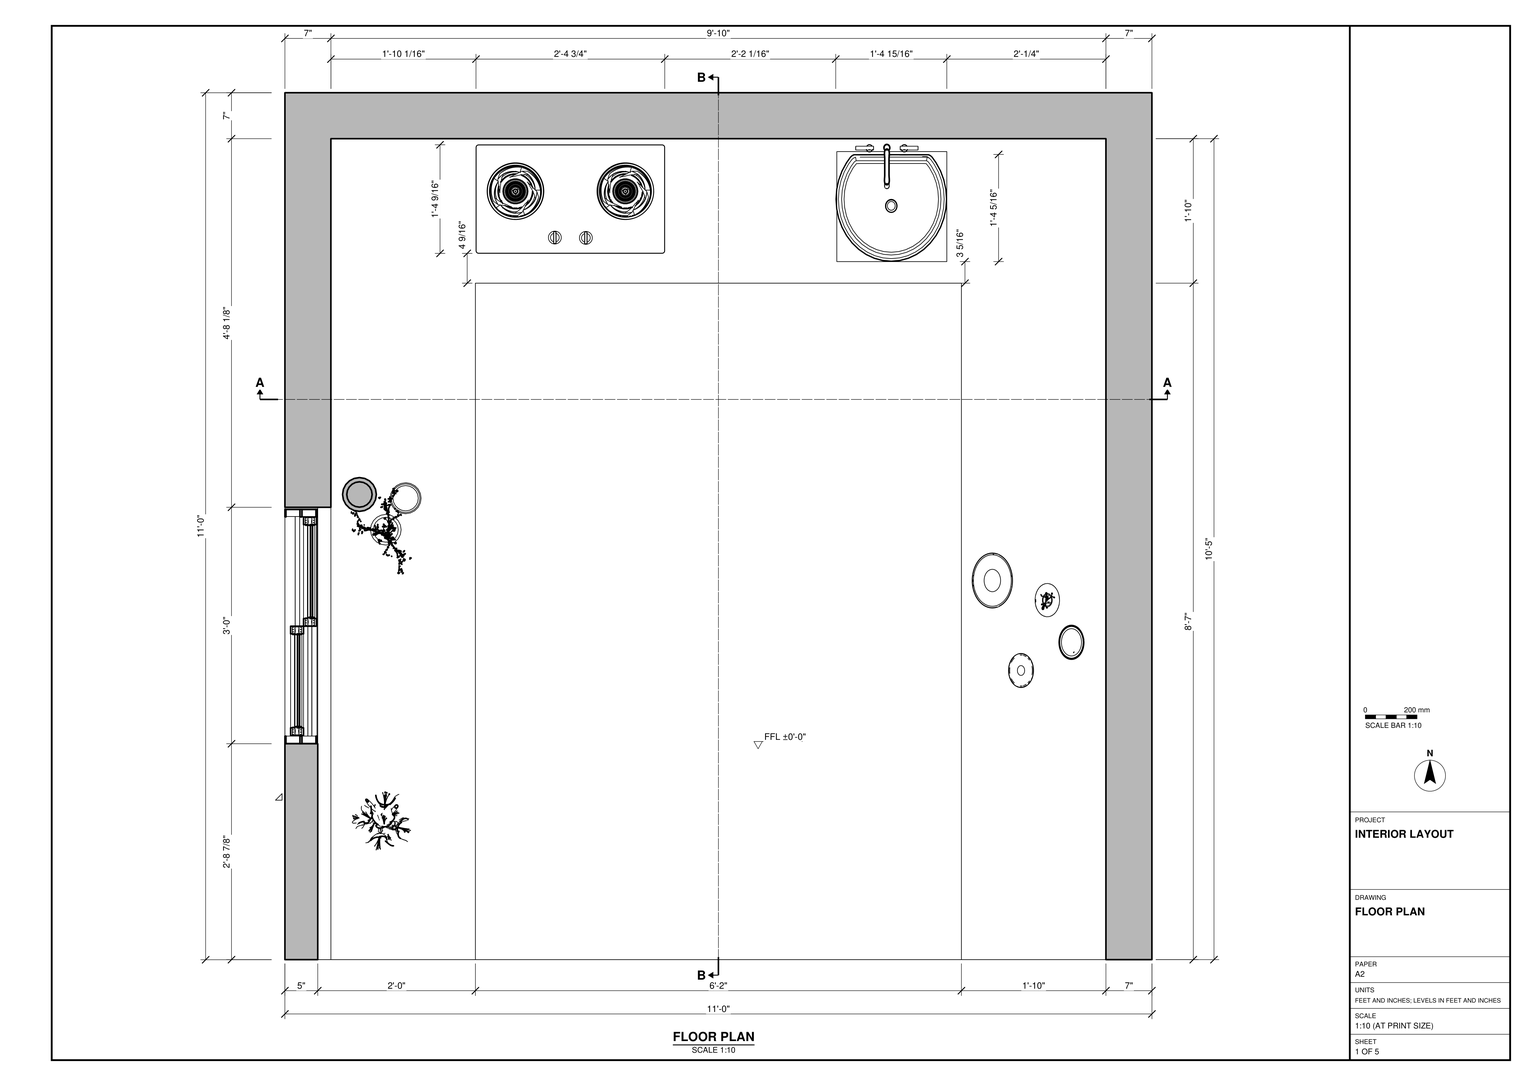
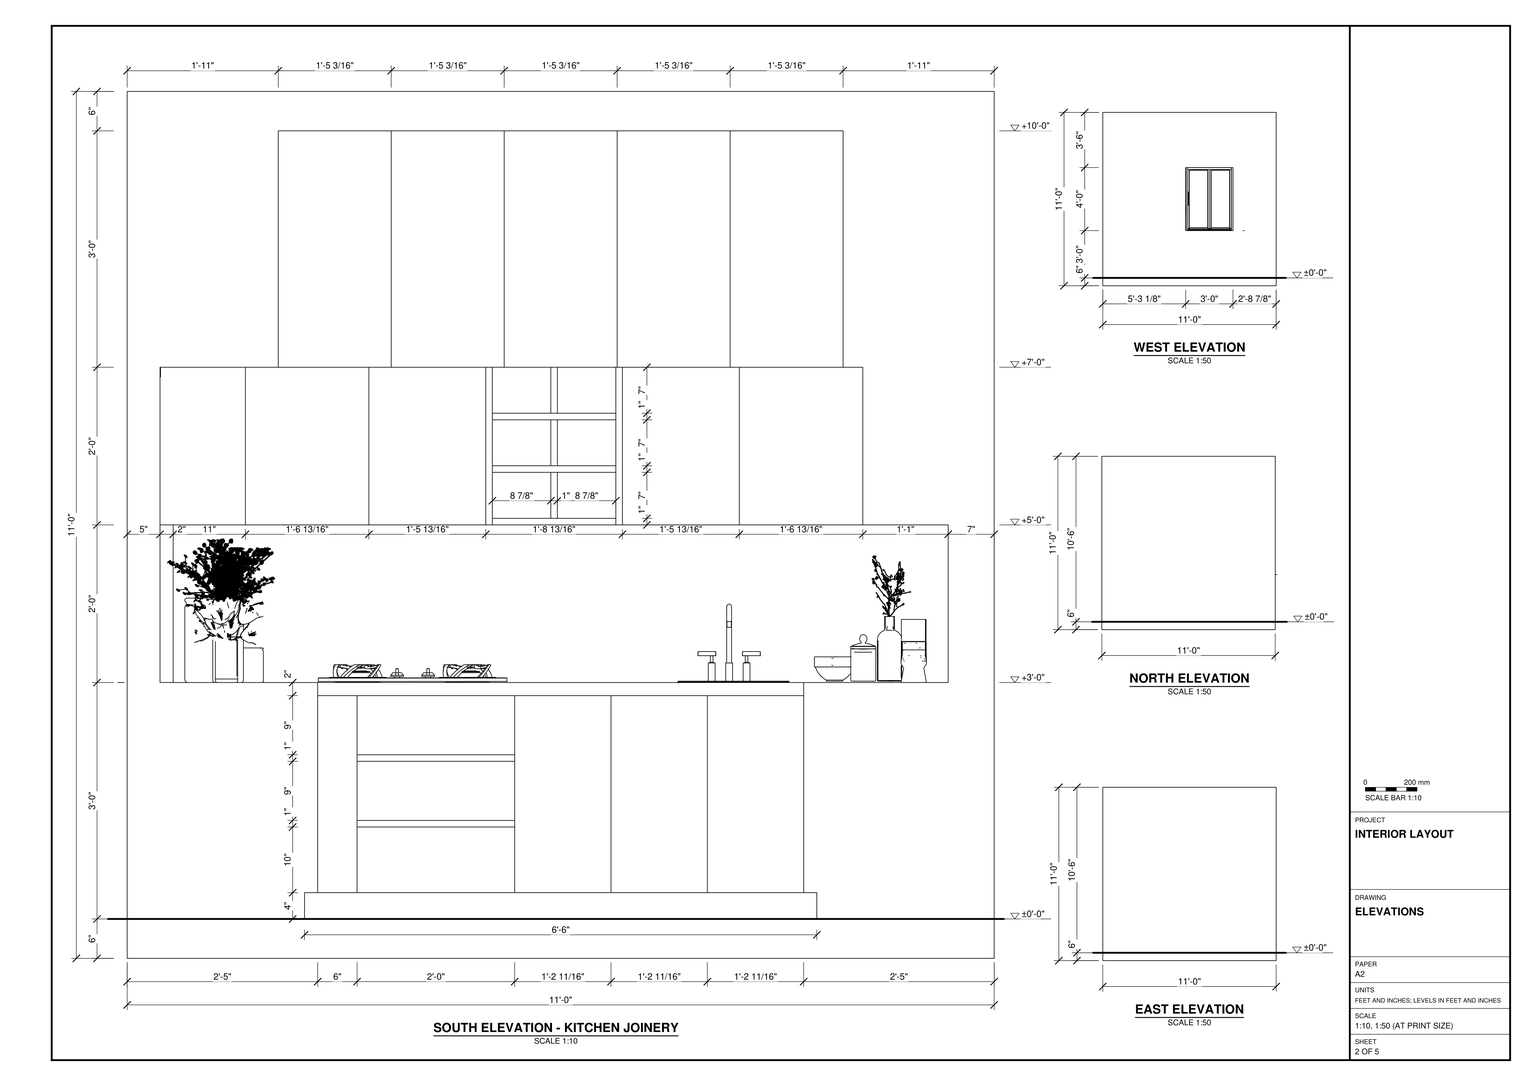
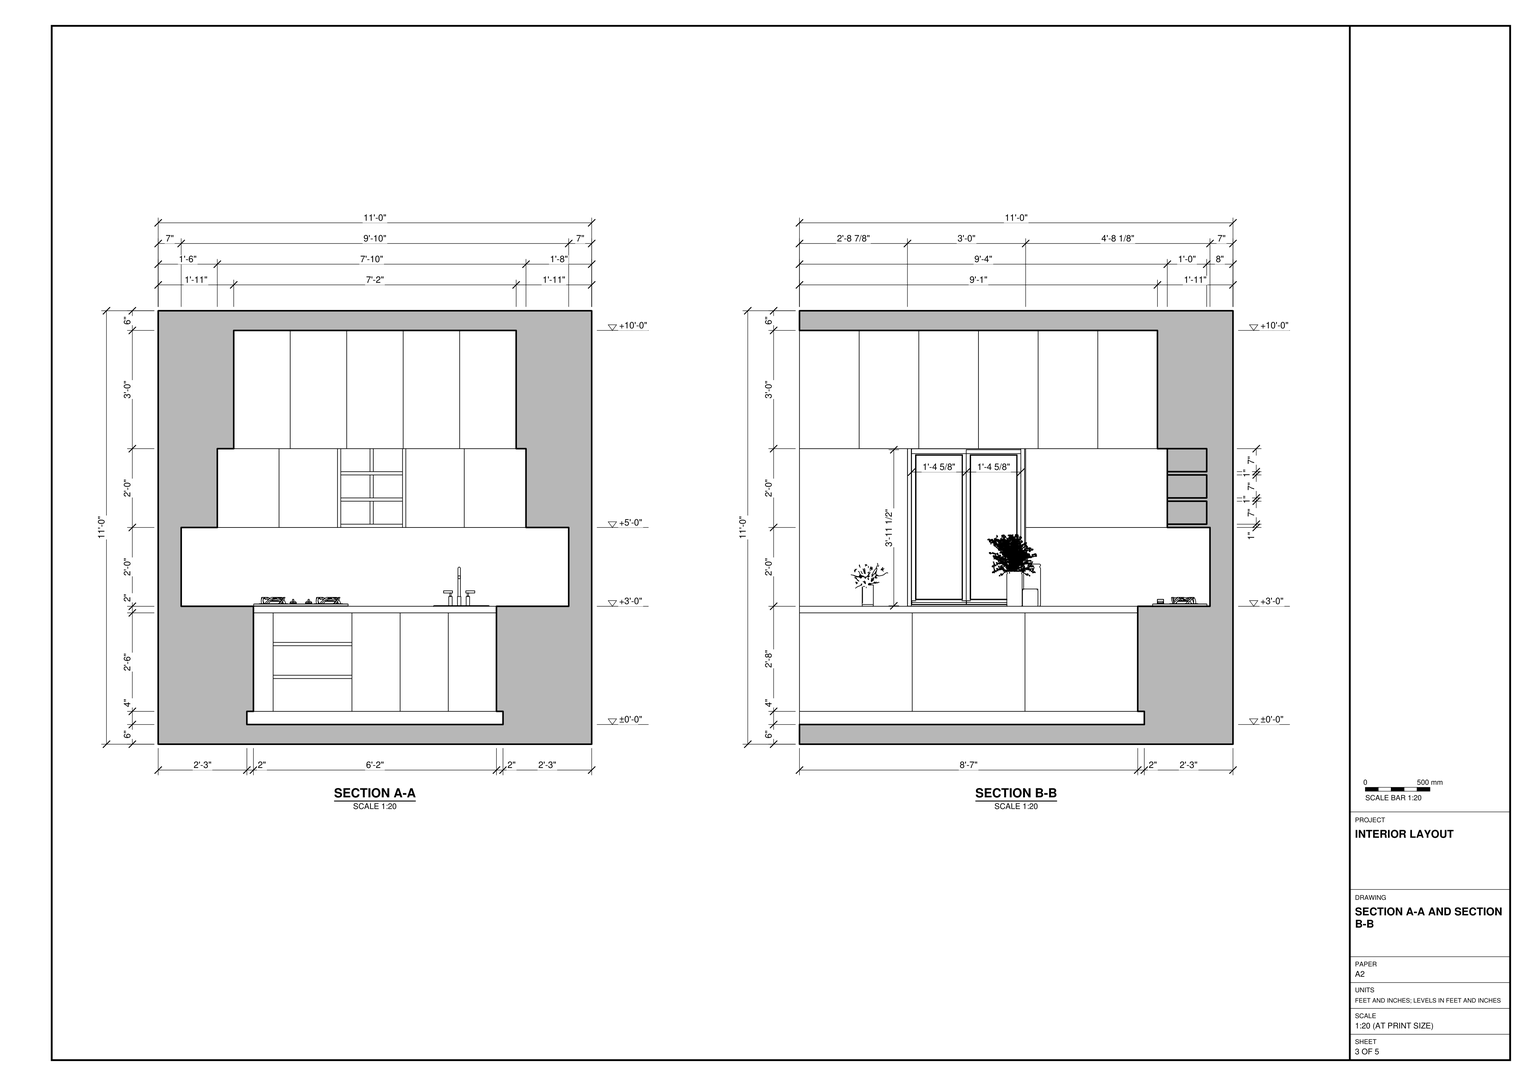
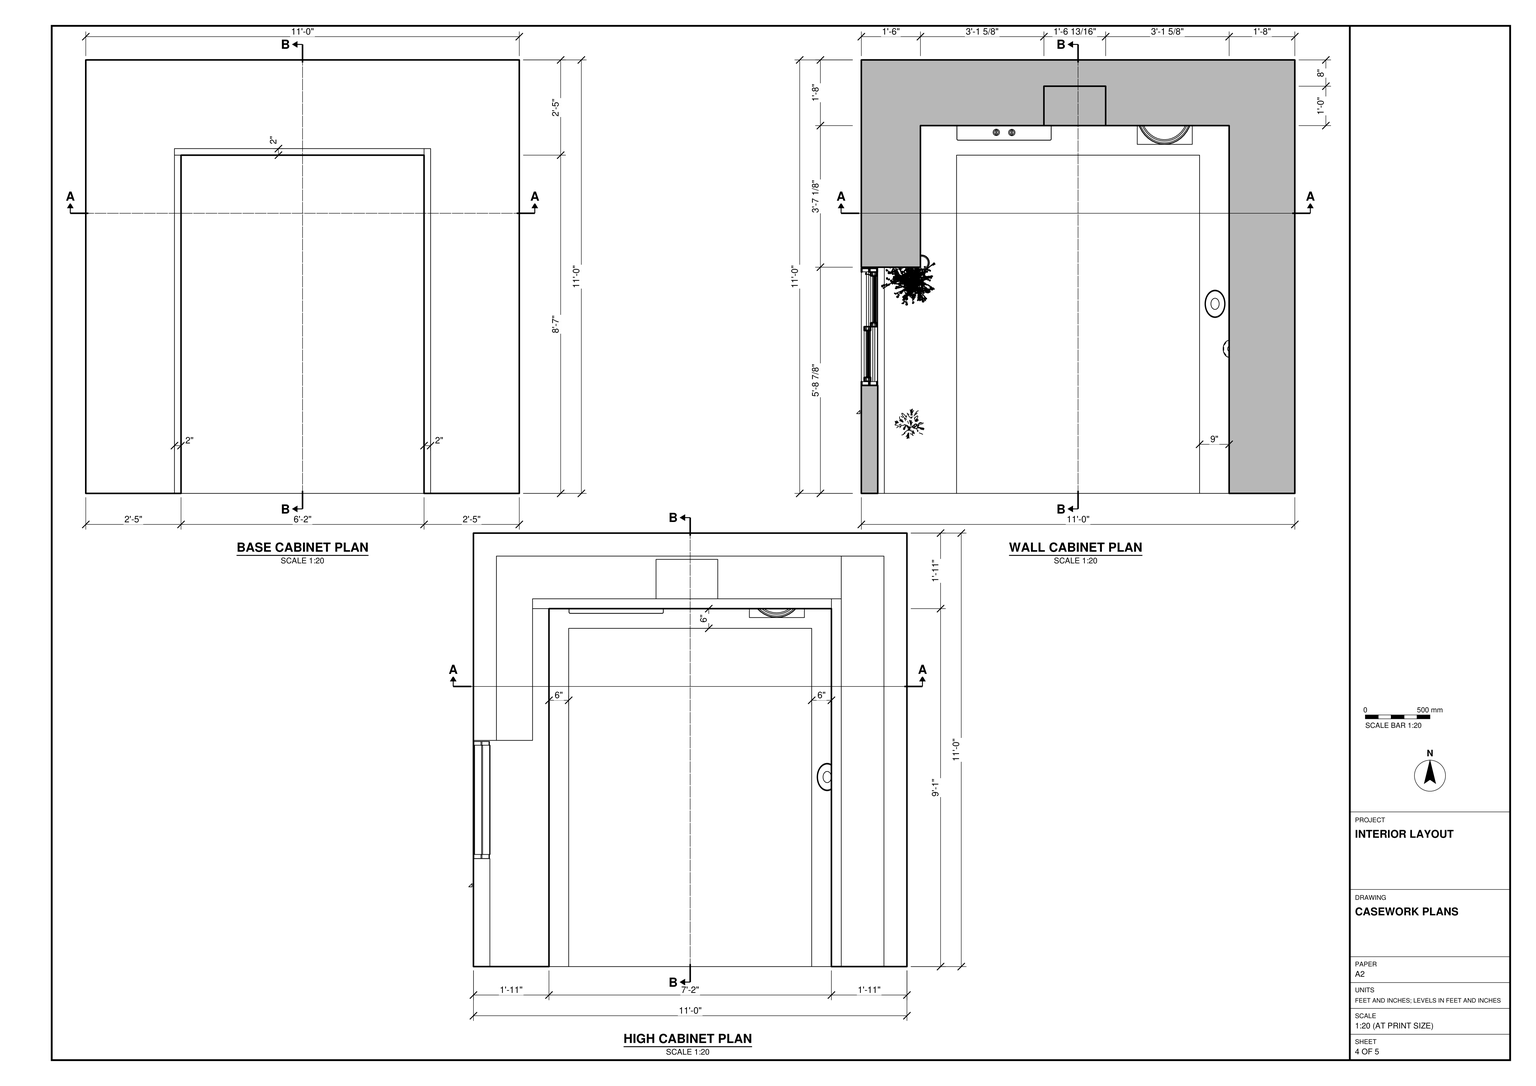
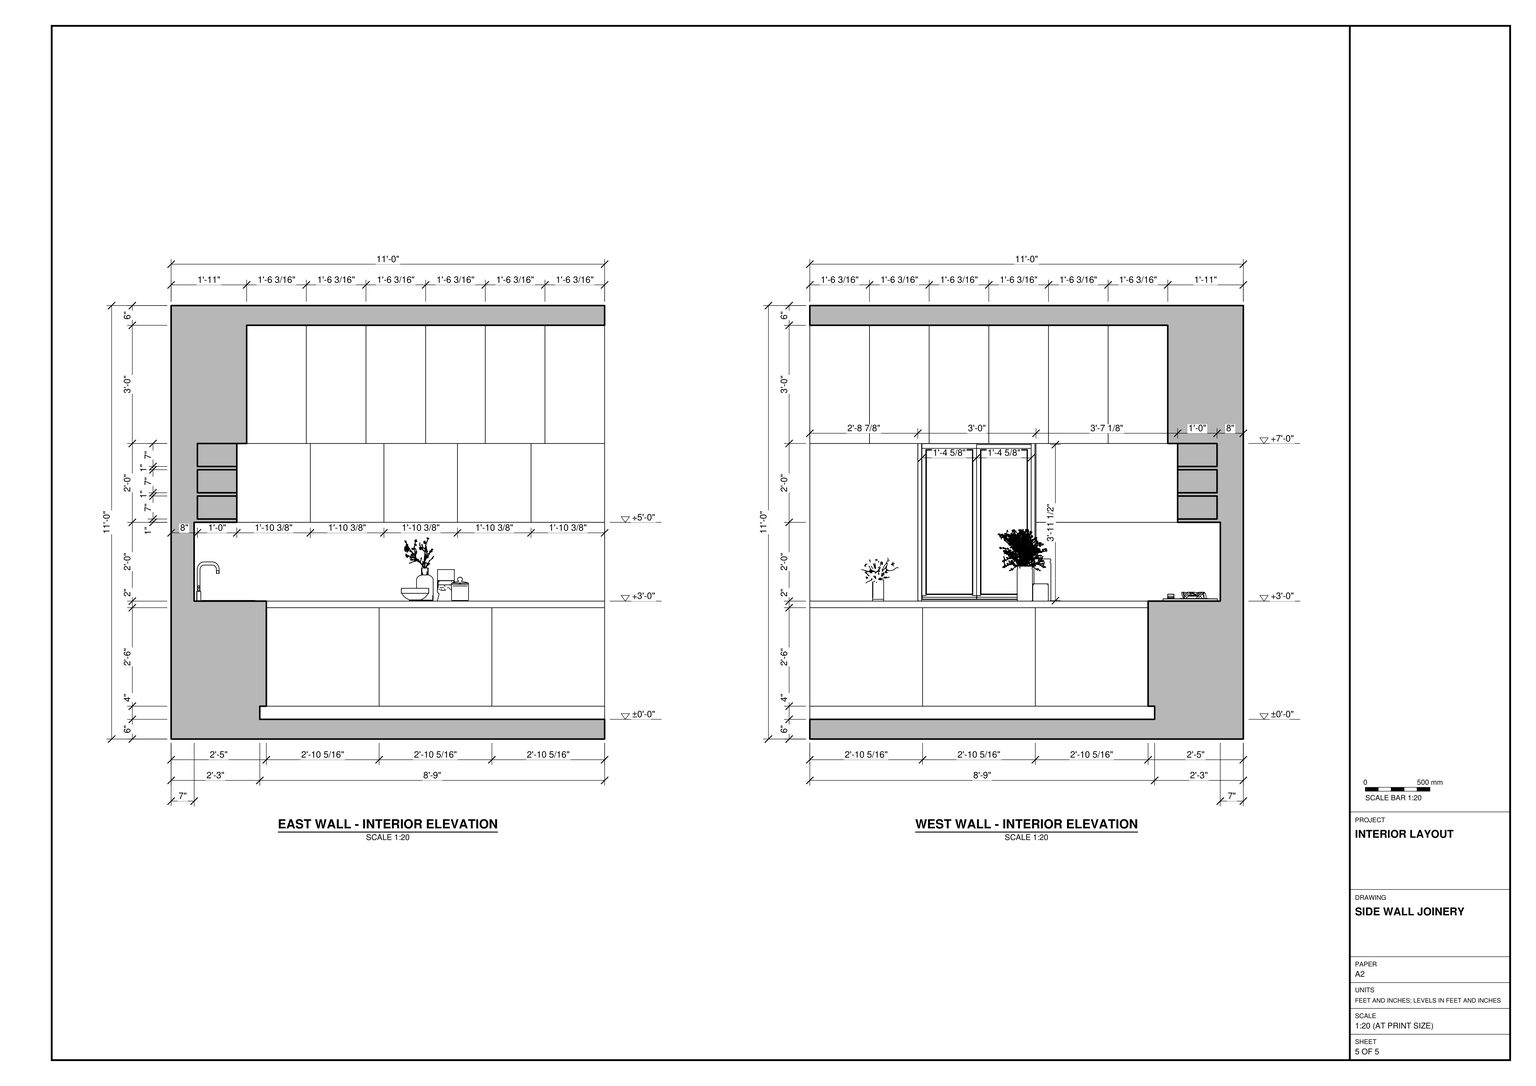
Build the kitchen interior in SketchUp using task_files/diagram_01.pdf. Work in feet and inches. The room is 11'-0" wide, 11'-0" deep and 11'-0" high overall, with the finished floor at ±0'-0". Model the floor slab, ceiling slab and three enclosing walls, leaving the front open as drawn. Follow the plan for the change in thickness along the west wall and fit the framed window into that wall.

Run the countertop around the back and both sides of the room, leaving the central aisle clear. Place the cooktop on the left of the back run and the sink and tap on the right. Use the joinery elevation for the drawer fronts, cabinet doors and open shelf compartments. Use the sections to set the countertop thickness, recessed toe spaces and the different depths of the two tiers of wall cabinets. Place the countertop objects in the positions shown in plan. Decor and loose items may be any suitable library components, for example from 3D Warehouse.

Keep the walls, slabs and individual joinery pieces in separate groups or components, and use components for repeated parts. Save one SketchUp model as output_files/u_shaped_kitchen_with_tiered_wall_cabinets.skp.

# SketchUp Ruby script. Lengths in inches.
U = 1.inch
M = Sketchup.active_model
def pt(a) = Geom::Point3d.new(a.map { |v| v * U })
def face(e, loops, mat)
  f = e.add_face(loops[0].map { |a| pt(a) })
  loops[1..].each { |l| e.add_face(l.map { |a| pt(a) }).erase! }
  f.material = f.back_material = mat if mat
  f
end
# faces: each face lists its corners as indices into pts; further lists are holes
def faces(e, pts, list, mat = nil) = list.each { |f| face(e, (f[0].is_a?(Array) ? f : [f]).map { |l| l.map { |i| pts[i] } }, mat) }
# xy, xz, yz: faces in a plane at the given z, y or x. An outline is a flat list of corners, or four numbers for a rectangle; further outlines are holes
def ring(l) = l.size == 4 ? [[l[0], l[1]], [l[2], l[1]], [l[2], l[3]], [l[0], l[3]]] : l.each_slice(2).to_a
def flat(e, list, mat, &to3) = list.each { |f| face(e, (f[0].is_a?(Array) ? f : [f]).map { |l| ring(l).map { |u, v| to3.(u, v) } }, mat) }
def xy(e, z, list, mat = nil) = flat(e, list, mat) { |x, y| [x, y, z] }
def xz(e, y, list, mat = nil) = flat(e, list, mat) { |x, z| [x, y, z] }
def yz(e, x, list, mat = nil) = flat(e, list, mat) { |y, z| [x, y, z] }
def lines(e, pts, list) = list.each { |a, b| e.add_line(pt(pts[a]), pt(pts[b])) }
# prism: a flat outline (further loops are holes) pulled along v
def prism(e, loops, v, mat = nil)
  f = face(e, loops, mat); d = Geom::Vector3d.new(v.map { |x| x * U })
  f.pushpull(f.normal.samedirection?(d) ? d.length : -d.length)
end
def box(e, o, s, mat = nil) = prism(e, [[o, [o[0] + s[0], o[1], o[2]], [o[0] + s[0], o[1] + s[1], o[2]], [o[0], o[1] + s[1], o[2]]]], [0, 0, s[2]], mat)
def at(x, y, z, deg = 0) = Geom::Transformation.translation(pt([x, y, z])) * Geom::Transformation.rotation(ORIGIN, Z_AXIS, deg.degrees)
def axes(o, x, y, z) = Geom::Transformation.new([*x, 0, *y, 0, *z, 0, *pt(o).to_a, 1])
def part(name) = M.definitions.add(name)
# library, detail: a bought-in or finely detailed component or shape, given as its bounding box
def library(name, o, s) = part(name).tap { |d| box(d.entities, o, s) }
def detail(e, o, s) = box(e.add_group.entities, o, s)
def put(e, d, t, mat = nil) = e.add_instance(d, t).tap { |i| i.material = mat if mat }
def group(e, t, mat = nil) = e.add_group.tap { |g| g.transformation = t; g.material = mat if mat }.entities
root = M.entities
M.materials.add("Aluminum_Anodized_DarkBrown").color = [41, 31, 11]
M.materials.add("Aluminum_Anodized_DarkGray").color = [62, 62, 62]
M.materials.add("Gold_24k").color = [35, 8, 0]
M.materials.add("Plastic_Metalic_Black").color = [8, 8, 8]
M.materials.add("VASO").color = [51, 51, 51]
M.materials.add("[0052_FloralWhite]").color = [255, 250, 240]
M.materials.add("[0053_Ivory]").color = [255, 255, 240]
M.materials.add("[Granite Dark Gray]").color = [69, 68, 68]
M.materials.add("[Metal_Corrogated_Shiny]1").color = [172, 139, 94]
M.materials.add("[Polished Concrete New]").color = [200, 200, 203]
M.materials.add("[Translucent Glass Sky Reflection]").color = [126, 138, 183]
M.materials["[Translucent Glass Sky Reflection]"].alpha = 0.52
M.materials.add("[Wood Veneer 01]").color = [120, 70, 37]
c1 = library("Gas hob burner",[0,0.01,0],[8.66,8.66,2.72])
c2 = part("Hob control knob")
xy(c2.entities,0,[[0.92,0.59,0.82,0.61,0.73,0.67,0.66,0.74,0.61,0.83,0.59,0.93,0.59,1.03,0.61,1.13,0.67,1.22,0.74,1.29,0.83,1.34,0.93,1.37,1.03,1.37,1.13,1.34,1.22,1.29,1.29,1.21,1.34,1.125,1.37,1.02,1.37,0.92,1.34,0.82,1.29,0.73,1.21,0.66,1.125,0.61,1.02,0.59]])
xy(c2.entities,0.2,[[[0.84,0,0.59,0.07,0.37,0.2,0.19,0.39,0.0625,0.61,0,0.86,0,1.12,0.07,1.36,0.2,1.58,0.39,1.76,0.61,1.89,0.86,1.95,1.12,1.95,1.36,1.88,1.58,1.75,1.76,1.57,1.89,1.34,1.95,1.1,1.95,0.84,1.88,0.59,1.75,0.37,1.57,0.19,1.34,0.0625,1.1,0],[0.92,0.59,1.02,0.59,1.125,0.61,1.21,0.66,1.29,0.73,1.34,0.82,1.37,0.92,1.37,1.02,1.34,1.125,1.29,1.21,1.22,1.29,1.13,1.34,1.03,1.37,0.93,1.37,0.83,1.34,0.74,1.29,0.67,1.22,0.61,1.13,0.59,1.03,0.59,0.93,0.61,0.83,0.66,0.74,0.73,0.67,0.82,0.61]]],"Aluminum_Anodized_DarkGray")
xy(c2.entities,0.39,[[[0.84,0,0.59,0.07,0.37,0.2,0.19,0.39,0.0625,0.61,0,0.86,0,1.12,0.07,1.36,0.2,1.58,0.39,1.76,0.61,1.89,0.86,1.95,1.12,1.95,1.36,1.88,1.58,1.75,1.76,1.57,1.89,1.34,1.95,1.1,1.95,0.84,1.88,0.59,1.75,0.37,1.57,0.19,1.34,0.0625,1.1,0],[0.05,0.78,1.91,1.17]],[0.05,0.78,1.91,1.17]])
xy(c2.entities,0.79,[[0.34,0.78,1.61,0.78,1.64,0.88,1.64,1.06,1.61,1.17,0.34,1.17,0.3125,1.07,0.3125,0.9]],"Aluminum_Anodized_DarkGray")
xy(c2.entities,0.79,[[0.88,0.3125,1.06,0.3125,1.23,0.36,1.38,0.44,1.5,0.5625,1.59,0.71,1.61,0.78,0.34,0.78,0.36,0.73,0.44,0.57,0.5625,0.45,0.71,0.36],[0.34,1.17,1.61,1.17,1.6,1.23,1.51,1.38,1.39,1.5,1.24,1.59,1.07,1.64,0.9,1.64,0.73,1.6,0.57,1.51,0.45,1.39,0.36,1.24]],"Plastic_Metalic_Black")
xy(c2.entities,1.42,[[0.09,0.82,1.87,1.14]],"Plastic_Metalic_Black")
xz(c2.entities,0,[[0.84,0.2,1.1,0.39]],"Aluminum_Anodized_DarkGray")
xz(c2.entities,0.59,[[0.92,0,1.02,0.2]],"Aluminum_Anodized_DarkGray")
xz(c2.entities,0.78,[[0.05,0.39,1.91,1.38]],"Aluminum_Anodized_DarkGray")
xz(c2.entities,1.17,[[0.05,0.39,1.91,1.38]],"Aluminum_Anodized_DarkGray")
xz(c2.entities,1.37,[[0.93,0,1.03,0.2]],"Aluminum_Anodized_DarkGray")
xz(c2.entities,1.95,[[0.86,0.2,1.12,0.39]],"Aluminum_Anodized_DarkGray")
yz(c2.entities,0,[[0.86,0.2,1.12,0.39]],"Aluminum_Anodized_DarkGray")
yz(c2.entities,0.05,[[0.78,0.39,1.17,1.38]],"Plastic_Metalic_Black")
yz(c2.entities,0.59,[[0.93,0,1.03,0.2]],"Aluminum_Anodized_DarkGray")
yz(c2.entities,1.37,[[0.92,0,1.02,0.2]],"Aluminum_Anodized_DarkGray")
yz(c2.entities,1.91,[[0.78,0.39,1.17,1.38]],"Plastic_Metalic_Black")
yz(c2.entities,1.95,[[0.84,0.2,1.1,0.39]],"Aluminum_Anodized_DarkGray")
p = [[0.73,0.67,0],[0.82,0.61,0],[0.82,0.61,0.2],[0.73,0.67,0.2],[0.92,0.59,0],[0.92,0.59,0.2],
  [1.02,0.59,0],[1.125,0.61,0],[1.125,0.61,0.2],[1.02,0.59,0.2],[1.21,0.66,0],[1.21,0.66,0.2],
  [0.61,0.83,0],[0.66,0.74,0],[0.66,0.74,0.2],[0.61,0.83,0.2],[1.29,0.73,0],[1.29,0.73,0.2],
  [1.34,0.82,0],[1.34,0.82,0.2],[0.59,0.93,0],[0.59,0.93,0.2],[1.37,0.92,0],[1.37,0.92,0.2],
  [0.61,1.13,0],[0.59,1.03,0],[0.59,1.03,0.2],[0.61,1.13,0.2],[1.37,1.02,0],[1.34,1.125,0],
  [1.34,1.125,0.2],[1.37,1.02,0.2],[0.67,1.22,0],[0.67,1.22,0.2],[1.29,1.21,0],[1.29,1.21,0.2],
  [0.74,1.29,0],[0.74,1.29,0.2],[1.22,1.29,0],[1.22,1.29,0.2],[0.83,1.34,0],[0.83,1.34,0.2],
  [0.93,1.37,0],[0.93,1.37,0.2],[1.13,1.34,0],[1.03,1.37,0],[1.03,1.37,0.2],[1.13,1.34,0.2],
  [0.59,0.07,0.39],[0.59,0.07,0.2],[0.84,0,0.2],[0.84,0,0.39],[1.1,0,0.39],[1.1,0,0.2],
  [1.34,0.0625,0.2],[1.34,0.0625,0.39],[0.37,0.2,0.39],[0.37,0.2,0.2],[1.57,0.19,0.2],[1.57,0.19,0.39],
  [0.19,0.39,0.39],[0.19,0.39,0.2],[1.75,0.37,0.2],[1.75,0.37,0.39],[0.0625,0.61,0.39],[0.0625,0.61,0.2],
  [1.88,0.59,0.2],[1.88,0.59,0.39],[0,0.86,0.39],[0,0.86,0.2],[1.95,0.84,0.2],[1.95,0.84,0.39],
  [0.07,1.36,0.39],[0.07,1.36,0.2],[0,1.12,0.2],[0,1.12,0.39],[1.95,1.1,0.39],[1.95,1.1,0.2],
  [1.89,1.34,0.2],[1.89,1.34,0.39],[1.76,1.57,0.2],[1.76,1.57,0.39],[0.2,1.58,0.39],[0.2,1.58,0.2],
  [0.39,1.76,0.39],[0.39,1.76,0.2],[1.58,1.75,0.2],[1.58,1.75,0.39],[0.61,1.89,0.39],[0.61,1.89,0.2],
  [1.36,1.88,0.2],[1.36,1.88,0.39],[0.86,1.95,0.39],[0.86,1.95,0.2],[1.12,1.95,0.2],[1.12,1.95,0.39],
  [0.88,0.3125,0.79],[0.71,0.36,0.79],[1.06,0.3125,0.79],[1.23,0.36,0.79],[0.5625,0.45,0.79],[1.38,0.44,0.79],
  [0.44,0.57,0.79],[1.5,0.5625,0.79],[0.36,0.73,0.79],[1.59,0.71,0.79],[0.34,0.78,0.79],[0.3125,0.9,0.79],
  [1.64,0.88,0.79],[1.61,0.78,0.79],[1.64,1.06,0.79],[0.3125,1.07,0.79],[0.34,1.17,0.79],[0.36,1.24,0.79],
  [1.6,1.23,0.79],[1.61,1.17,0.79],[0.45,1.39,0.79],[1.51,1.38,0.79],[0.57,1.51,0.79],[1.39,1.5,0.79],
  [0.73,1.6,0.79],[1.24,1.59,0.79],[0.9,1.64,0.79],[1.07,1.64,0.79],[0.09,0.82,1.42],[0.09,1.14,1.42],
  [0.05,1.17,1.38],[0.05,0.78,1.38],[1.87,0.82,1.42],[1.91,0.78,1.38],[1.87,1.14,1.42],[1.91,1.17,1.38]]
faces(c2.entities,p,[[0,1,2,3],[1,4,5,2],[6,7,8,9],[7,10,11,8],[12,13,14,15],[13,0,3,14],[10,16,17,11],[16,18,19,17],
  [20,12,15,21],[18,22,23,19],[24,25,26,27],[28,29,30,31],[32,24,27,33],[29,34,35,30],[36,32,33,37],[34,38,39,35],
  [40,36,37,41],[42,40,41,43],[44,45,46,47],[38,44,47,39],[48,49,50,51],[52,53,54,55],[56,57,49,48],[55,54,58,59],
  [60,61,57,56],[59,58,62,63],[64,65,61,60],[63,62,66,67],[68,69,65,64],[67,66,70,71],[72,73,74,75],[76,77,78,79],
  [79,78,80,81],[82,83,73,72],[84,85,83,82],[81,80,86,87],[88,89,85,84],[87,86,90,91],[92,93,89,88],[91,90,94,95],
  [124,125,126,127],[128,124,127,129],[130,128,129,131],[131,126,125,130]],"Aluminum_Anodized_DarkGray")
faces(c2.entities,p,[[51,96,97,48],[52,98,96,51],[55,99,98,52],[48,97,100,56],[59,101,99,55],[100,102,60,56],[63,103,101,59],[102,104,64,60],
  [63,67,105,103],[106,107,68,64,104],[67,71,108,109,105],[71,76,110,108],[107,111,75,68],[112,113,72,75,111],[76,79,114,115,110],[113,116,82,72],
  [79,81,117,114],[82,116,118,84],[81,87,119,117],[84,118,120,88],[91,121,119,87],[88,120,122,92],[92,122,123,95],[95,123,121,91]],"Gold_24k")
c3 = library("GasStove_E",[0,-1.18,0],[28.74,16.53,0.59])
c4 = library("Cylinder01",[-250,-263.26,0],[500,428.9,60.12])
c5 = library("Cylinder02",[-26.76,-32.04,0],[53.52,53.22,4.76])
c6 = library("Cylinder03",[-17.61,-22.94,0],[35.22,35.03,2.22])
c7 = library("Line01",[-11.86,89.7,-318.58],[30.8,179.84,332.63])
c8 = library("建立群組\#1",[0,0,0],[80.82,30.8,167.59])
c9 = part("建立群組\#2")
put(c9.entities,c7,at(136.97,-89.7,318.58))
put(c9.entities,c8,at(0,146.85,0))
put(c9.entities,c8,axes([281.01,146.85,0],[-1,0,0],[0,1,0],[0,0,1]))
c10 = part("skp712A")
put(c10.entities,c4,at(0,0,0))
put(c10.entities,c5,at(0,-34.98,0))
put(c10.entities,c6,at(0,-34.65,0))
put(c10.entities,c9,at(-160.32,28.05,-4.6))
c11 = library("Lily Flower",[-11.23,-7.61,-0.93],[19.43,20.89,23.03])
c12 = library("FF_Model_ID10967_2_VA004_rustic_vases_PR_FMH",[-13.24,-7.65,0],[22.68,26.4,28.35])
c13 = library("Agrupar\#44",[-6.1,-5.77,2.8],[28.99,25.99,16.38])
c14 = library("Group\#21",[0,0,0],[39.41,1.97,87.22])
c15 = part("Group\#16")
xy(c15.entities,0,[[-9.26,-0.47,78.74,4.41]])
xy(c15.entities,0.08,[[-9.26,-0.31,78.74,1.8125],[-9.26,2.125,78.74,4.25]])
xy(c15.entities,2.76,[[-9.26,-0.47,78.74,-0.31],[-9.26,1.8125,78.74,2.125],[-9.26,4.25,78.74,4.41]])
xz(c15.entities,-0.47,[[-9.26,0,78.74,2.76]])
xz(c15.entities,-0.31,[[-9.26,0.08,78.74,2.76]])
xz(c15.entities,1.8125,[[-9.26,0.08,78.74,2.76]])
xz(c15.entities,2.125,[[-9.26,0.08,78.74,2.76]])
xz(c15.entities,4.25,[[-9.26,0.08,78.74,2.76]])
xz(c15.entities,4.41,[[-9.26,0,78.74,2.76]])
yz(c15.entities,-9.26,[[-0.47,0,-0.47,2.76,-0.31,2.76,-0.31,0.08,1.8125,0.08,1.8125,2.76,2.125,2.76,2.125,0.08,4.25,0.08,4.25,2.76,4.41,2.76,4.41,0]])
yz(c15.entities,78.74,[[-0.47,0,-0.31,2.76],[-0.31,0,1.8125,0.08],[1.8125,0,2.125,2.76],[2.125,0,4.25,0.08],[4.25,0,4.41,2.76]])
p = [[0.16,2.125,0.08],[0.16,1.8125,0.08]]
lines(c15.entities,p,[[0,1]])
c16 = library("Group\#20",[0,0,0],[0.83,1.4,0.31])
c17 = library("Group\#19",[0,0,0],[0.83,1.4,0.31])
c18 = library("Group\#32",[0,0,0],[13.84,16.39,35.5])
c19 = library("Group\#35",[0,0,0],[4.21,4.21,8.92])
c20 = library("Group\#33",[0,0,0],[6.71,6.71,3.4375])
c21 = library("Group\#34",[0,0,0],[3.56,3.56,5.63])
xy(root,0,[[0,0,132,132]])
xy(root,6,[[27,0,105,105]],"[Polished Concrete New]")
xy(root,10,[[27,103,103,105]])
xy(root,10,[[27,0,29,103],[103,0,105,105]],"[0052_FloralWhite]")
xy(root,32,[[84.03,106.29,100.78,123.04]],"[Granite Dark Gray]")
xy(root,42,[[0,32.875,5,68.875]])
xy(root,42,[[5,0,7,68.875]],"[0052_FloralWhite]")
xy(root,42,[[[7,0,29,0,29,103,103,103,103,0,125,0,125,125,7,125],[84.03,106.29,100.78,123.04]]],"[Granite Dark Gray]")
xy(root,66,[[112,0,125,125],[7,68.875,7,125,112,125,112,112,18,112,18,68.875]],"[Wood Veneer 01]")
xy(root,67,[[55.6,112,74.4,124]])
xy(root,74,[[55.6,112,74.4,124]])
xy(root,75,[[55.6,112,74.4,124]])
xy(root,82,[[55.6,112,74.4,124]])
xy(root,83,[[55.6,112,74.4,124]])
xy(root,90,[[55.6,112,74.4,124]])
xy(root,90,[[5,0,5,32.875,0,32.875,0,68.875,18,68.875,18,109,23,109,23,0],[109,0,112,112],[18,109,109,112]],"[0052_FloralWhite]")
xy(root,126,[[23,0,109,109]])
xy(root,132,[[0,0,132,132]],"[0052_FloralWhite]")
xz(root,0,[[[0,0,132,132],[27,6,27,10,29,10,29,42,5,42,5,90,23,90,23,126,109,126,109,90,112,90,112,66,125,66,125,42,103,42,103,10,105,10,105,6]]],"[0052_FloralWhite]")
xz(root,32.875,[[0,42,5,90]])
xz(root,68.875,[[0,42,7,66]])
xz(root,68.875,[[0,66,18,90]],"[Wood Veneer 01]")
xz(root,103,[[29,10,35,40],[35,10,59,20],[59,10,73.67,40],[73.67,10,88.33,40],[88.33,10,103,40],
  [35,21,59,30],[35,31,59,40]],"[0052_FloralWhite]")
xz(root,103,[[29,40,103,42]],"[Granite Dark Gray]")
xz(root,103,[[35,20,59,21],[35,30,59,31]],"[Wood Veneer 01]")
xz(root,105,[[27,6,105,10]],"[Wood Veneer 01]")
xz(root,106.29,[[84.03,32,100.78,42]],"[Granite Dark Gray]")
xz(root,109,[[23,90,40.2,126],[40.2,90,57.4,126],[57.4,90,74.6,126],[74.6,90,91.8,126],[91.8,90,109,126]],"[0052_FloralWhite]")
xz(root,112,[[55.6,67,64.5,74],[65.5,67,74.4,74],[55.6,75,64.5,82],[65.5,75,74.4,82],[55.6,83,64.5,90],
  [65.5,83,74.4,90]],"[Translucent Glass Sky Reflection]")
xz(root,112,[[18,66,36.8,90],[36.8,66,54.6,90],[54.6,66,55.6,90],[55.6,66,74.4,67],[74.4,66,75.4,90],
  [75.4,66,93.2,90],[93.2,66,112,90],[64.5,67,65.5,74],[55.6,74,74.4,75],[64.5,75,65.5,82],
  [55.6,82,74.4,83],[64.5,83,65.5,90]],"[Wood Veneer 01]")
xz(root,123.04,[[84.03,32,100.78,42]],"[Granite Dark Gray]")
xz(root,124,[[55.6,67,74.4,74],[55.6,75,74.4,82],[55.6,83,74.4,90]])
xz(root,125,[[7,42,125,66]],"[Polished Concrete New]")
xz(root,132,[[0,0,132,132]],"[0053_Ivory]")
yz(root,0,[[[0,0,132,132],[32.875,42,68.875,90]]],"[0053_Ivory]")
yz(root,5,[[0,42,32.875,90]],"[0052_FloralWhite]")
yz(root,7,[[68.875,42,125,66]],"[Polished Concrete New]")
yz(root,18,[[68.875,66,112,90]],"[Wood Veneer 01]")
yz(root,23,[[0,90,18.17,126],[18.17,90,36.33,126],[36.33,90,54.5,126],[54.5,90,72.67,126],[72.67,90,90.83,126],
  [90.83,90,109,126]],"[0052_FloralWhite]")
yz(root,27,[[0,6,105,10]],"[Wood Veneer 01]")
yz(root,29,[[0,10,34.33,40],[34.33,10,68.67,40],[68.67,10,103,40]],"[0052_FloralWhite]")
yz(root,29,[[0,40,103,42]],"[Granite Dark Gray]")
yz(root,55.6,[[112,67,124,74],[112,75,124,82],[112,83,124,90]])
yz(root,74.4,[[112,67,124,74],[112,75,124,82],[112,83,124,90]])
yz(root,84.03,[[106.29,32,123.04,42]],"[Granite Dark Gray]")
yz(root,100.78,[[106.29,32,123.04,42]],"[Granite Dark Gray]")
yz(root,103,[[0,10,34.33,40],[34.33,10,68.67,40],[68.67,10,103,40]],"[0052_FloralWhite]")
yz(root,103,[[0,40,103,42]],"[Granite Dark Gray]")
yz(root,105,[[0,6,105,10]],"[Wood Veneer 01]")
yz(root,109,[[0,90,18.17,126],[18.17,90,36.33,126],[36.33,90,54.5,126],[54.5,90,72.67,126],[72.67,90,90.83,126],
  [90.83,90,109,126]],"[0052_FloralWhite]")
yz(root,112,[[0,66,22.4,90],[22.4,66,44.8,90],[44.8,66,67.2,90],[67.2,66,89.6,90],[89.6,66,112,90]],"[Wood Veneer 01]")
yz(root,125,[[0,42,125,66]],"[Polished Concrete New]")
yz(root,132,[[0,0,132,132]],"[0053_Ivory]")
p = [[40.2,109.6,90],[40.2,109.6,126],[57.4,110.2,90],[57.4,110.2,126],[74.6,110.8,90],[74.6,110.8,126],
  [91.8,111.4,90],[91.8,111.4,126],[-1.4375,24.28,42],[-0.4375,24.28,42],[-0.4375,25.28,42],[109,112,90],
  [109,112,126]]
lines(root,p,[[0,1],[2,3],[4,5],[6,7],[8,9],[9,10],[10,8],[11,12]])
put(root,c1,at(30.77,112.66,42))
put(root,c2,at(42.07,108.97,42.71,90))
put(root,c2,at(46.8,108.92,42.71,90))
put(root,c3,at(29.09,108.72,42.12))
put(root,c1,at(47.5,112.66,42))
put(root,c10,axes([92.32,116.3,39.58],[0.03383,0,0],[0,0.03805,0],[0,0,0.0438]))
put(root,c11,axes([16.27,19.51,42.53],[0.57,0,0],[0,0.57,0],[0,0,0.57]))
put(root,c12,axes([12.24,67.4,42],[-0.00008,-0.4536,0],[0.4536,-0.00008,0],[0,0,0.4536]),"[Metal_Corrogated_Shiny]1")
put(root,c13,at(6.11,57.27,45.54),"VASO")
put(root,c14,axes([0.87,50.79,42.14],[0,-0.42249,0],[1,0,0],[0,0,0.54494]),"Aluminum_Anodized_DarkBrown")
put(root,c14,axes([2.83,67.42,42.14],[0,-0.42249,0],[1,0,0],[0,0,0.54494]),"Aluminum_Anodized_DarkBrown")
g1 = group(root,at(0.87,85.09,42.47),"Aluminum_Anodized_DarkBrown")
prism(g1,[[[1.375,-17.61,0],[2.64,-17.61,0],[2.62,-17.61,-0.05],[2.64,-17.61,-0.1],[2.68,-17.61,-0.15],[2.75,-17.61,-0.19],[2.84,-17.61,-0.21],[2.93,-17.61,-0.22],[3.03,-17.61,-0.21],[3.11,-17.61,-0.19],[3.18,-17.61,-0.15],[3.22,-17.61,-0.1],[3.24,-17.61,-0.05],[3.23,-17.61,0],[4.02,-17.61,0],[4.02,-17.61,-0.43],[-0.87,-17.61,-0.43],[-0.87,-17.61,0],[0.7,-17.61,0],[0.69,-17.61,-0.06],[0.72,-17.61,-0.11],[0.77,-17.61,-0.16],[0.84,-17.61,-0.2],[0.9375,-17.61,-0.23],[1.04,-17.61,-0.24],[1.14,-17.61,-0.23],[1.24,-17.61,-0.2],[1.3125,-17.61,-0.16],[1.36,-17.61,-0.11],[1.39,-17.61,-0.06]]],[0,-33.43,0])
g2 = group(root,at(4.61,67.41,90),"Aluminum_Anodized_DarkBrown")
xy(g2,-1.5,[[-4.41,-33.27,-4.25,0],[-2.125,-33.27,-1.8125,0],[0.31,-33.27,0.47,0]])
xy(g2,-0.04,[[-4.25,-33.27,-2.125,0],[-1.8125,-33.27,0.31,0]])
xy(g2,0,[[-4.41,-33.27,0.47,0]])
xz(g2,-33.27,[[-4.41,-1.5,-4.25,0],[-2.125,-1.5,-1.8125,0],[0.31,-1.5,0.47,0],[-4.25,-0.04,-2.125,0],[-1.8125,-0.04,0.31,0]])
xz(g2,0,[[-4.41,-1.5,-4.25,0],[-2.125,-1.5,-1.8125,0],[0.31,-1.5,0.47,0],[-4.25,-0.04,-2.125,0],[-1.8125,-0.04,0.31,0]])
yz(g2,-4.41,[[-33.27,-1.5,0,0]])
yz(g2,-4.25,[[-33.27,-1.5,0,-0.04]])
yz(g2,-2.125,[[-33.27,-1.5,0,-0.04]])
yz(g2,-1.8125,[[-33.27,-1.5,0,-0.04]])
yz(g2,0.31,[[-33.27,-1.5,0,-0.04]])
yz(g2,0.47,[[-33.27,-1.5,0,0]])
p = [[-2.125,-0.07,-0.04],[-1.8125,-0.07,-0.04]]
lines(g2,p,[[0,1]])
put(root,c15,axes([4.41,32.875,84.95],[0,0,-0.54494],[-1,0,0],[0,0.42249,0]),"Aluminum_Anodized_DarkBrown")
put(root,c15,axes([0.47,68.57,84.95],[0,0,-0.54494],[1,0,0],[0,-0.42249,0]),"Aluminum_Anodized_DarkBrown")
put(root,c16,axes([1.4375,66.82,63.87],[0,-0.42249,0],[1,0,0],[0,0,0.54494]),"Aluminum_Anodized_DarkBrown")
put(root,c17,axes([1.4375,66.82,69.1875],[0,-0.42249,0],[1,0,0],[0,0,0.54494]),"Aluminum_Anodized_DarkBrown")
g3 = group(root,at(1.26,67.34,61.29),"Aluminum_Anodized_DarkBrown")
box(g3,[0,-0.73,0],[0.2,0.56,10.0625])
put(root,c18,axes([121.04,56.31,42.21],[-0.3084,0.46418,0],[-0.34131,-0.41942,0],[0,0,0.5382]))
put(root,c19,axes([117.82,50.95,42],[0,-1.2512,0],[0.92,0,0],[0,0,1.0764]))
put(root,c20,axes([104.62,61.93,42.21],[0,-1.2512,0],[0.92,0,0],[0,0,1.0764]))
put(root,c21,axes([110.16,46.63,42.21],[0,-1.4639,0],[1.0764,0,0],[0,0,1.25939]))
